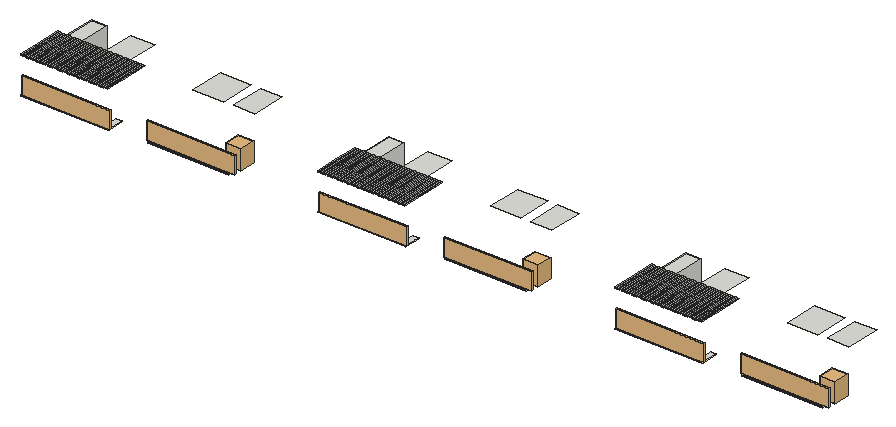
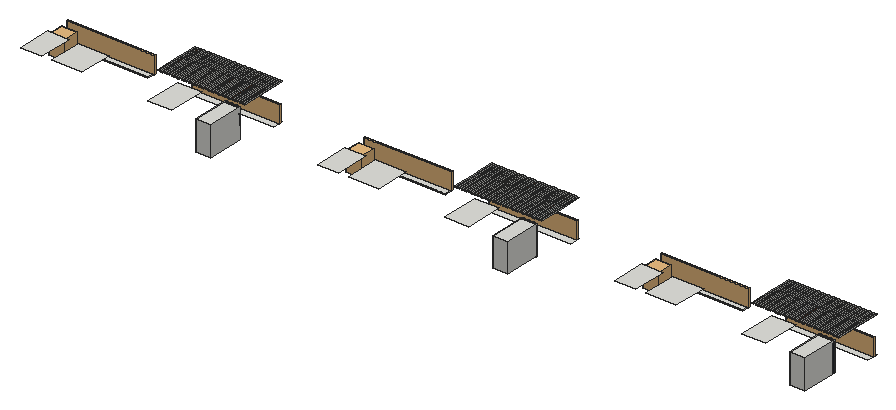
# SketchUp Ruby script. Lengths in inches.
U = 1.inch
M = Sketchup.active_model
def pt(a) = Geom::Point3d.new(a.map { |v| v * U })
def face(e, loops, mat)
  f = e.add_face(loops[0].map { |a| pt(a) })
  loops[1..].each { |l| e.add_face(l.map { |a| pt(a) }).erase! }
  f.material = f.back_material = mat if mat
  f
end
# faces: each face lists its corners as indices into pts; further lists are holes
def faces(e, pts, list, mat = nil) = list.each { |f| face(e, (f[0].is_a?(Array) ? f : [f]).map { |l| l.map { |i| pts[i] } }, mat) }
# xy, xz, yz: faces in a plane at the given z, y or x. An outline is a flat list of corners, or four numbers for a rectangle; further outlines are holes
def ring(l) = l.size == 4 ? [[l[0], l[1]], [l[2], l[1]], [l[2], l[3]], [l[0], l[3]]] : l.each_slice(2).to_a
def flat(e, list, mat, &to3) = list.each { |f| face(e, (f[0].is_a?(Array) ? f : [f]).map { |l| ring(l).map { |u, v| to3.(u, v) } }, mat) }
def xy(e, z, list, mat = nil) = flat(e, list, mat) { |x, y| [x, y, z] }
def xz(e, y, list, mat = nil) = flat(e, list, mat) { |x, z| [x, y, z] }
def yz(e, x, list, mat = nil) = flat(e, list, mat) { |y, z| [x, y, z] }
def lines(e, pts, list) = list.each { |a, b| e.add_line(pt(pts[a]), pt(pts[b])) }
# prism: a flat outline (further loops are holes) pulled along v
def prism(e, loops, v, mat = nil)
  f = face(e, loops, mat); d = Geom::Vector3d.new(v.map { |x| x * U })
  f.pushpull(f.normal.samedirection?(d) ? d.length : -d.length)
end
def box(e, o, s, mat = nil) = prism(e, [[o, [o[0] + s[0], o[1], o[2]], [o[0] + s[0], o[1] + s[1], o[2]], [o[0], o[1] + s[1], o[2]]]], [0, 0, s[2]], mat)
def at(x, y, z, deg = 0) = Geom::Transformation.translation(pt([x, y, z])) * Geom::Transformation.rotation(ORIGIN, Z_AXIS, deg.degrees)
def axes(o, x, y, z) = Geom::Transformation.new([*x, 0, *y, 0, *z, 0, *pt(o).to_a, 1])
def part(name) = M.definitions.add(name)
# library, detail: a bought-in or finely detailed component or shape, given as its bounding box
def library(name, o, s) = part(name).tap { |d| box(d.entities, o, s) }
def detail(e, o, s) = box(e.add_group.entities, o, s)
def put(e, d, t, mat = nil) = e.add_instance(d, t).tap { |i| i.material = mat if mat }
def group(e, t, mat = nil) = e.add_group.tap { |g| g.transformation = t; g.material = mat if mat }.entities
root = M.entities
M.materials.add("Wine2").color = [0, 0, 0]
M.materials["Wine2"].alpha = 0
M.materials.add("[0130_Gainsboro]").color = [39, 45, 50]
M.materials.add("[Wood Veneer 01]").color = [51, 28, 15]
c1 = library("plant (1)",[-35.72,-28.42,0],[66.31,67.39,84.38])
c2 = library("Glass Railing",[0,0,0],[139.5,4.76,42])
c3 = part("Group\#55")
xy(c3.entities,0,[[0,-0.98,43.07,0],[0,0,43.07,1.4]],"[0130_Gainsboro]")
xy(c3.entities,0.3,[[0.3,-1.43,42.77,-0.98]],"[0130_Gainsboro]")
xy(c3.entities,2.95,[[2.95,-1.43,40.12,-0.63],[2.95,-0.63,40.12,0],[2.95,0,40.12,0.64],[2.95,0.64,40.12,1.4]],"[0130_Gainsboro]")
xy(c3.entities,3.54,[[3.54,-0.63,39.53,0],[3.54,0,39.53,0.64]],"[0130_Gainsboro]")
xy(c3.entities,111.8125,[[3.54,-0.63,39.53,0],[3.54,0,39.53,0.64]],"[0130_Gainsboro]")
xy(c3.entities,112.4,[[2.95,-1.43,40.12,-0.63],[2.95,-0.63,40.12,0],[2.95,0,40.12,0.64],[2.95,0.64,40.12,1.4]],"[0130_Gainsboro]")
xy(c3.entities,115.05,[[0.3,-1.43,42.77,-0.98]],"[0130_Gainsboro]")
xy(c3.entities,115.35,[[0,-0.98,43.07,0],[0,0,43.07,1.4]],"[0130_Gainsboro]")
xz(c3.entities,-1.43,[[[0.3,0.3,42.77,115.05],[2.95,2.95,40.12,112.4]]],"[Wood Veneer 01]")
xz(c3.entities,-0.98,[[[0,0,43.07,115.35],[0.3,0.3,42.77,115.05]]],"[0130_Gainsboro]")
xz(c3.entities,-0.63,[[[2.95,2.95,40.12,112.4],[3.54,3.54,39.53,111.8125]]],"[0130_Gainsboro]")
xz(c3.entities,0,[[3.54,3.54,39.53,111.8125]],"Wine2")
xz(c3.entities,0,[[[0,0,43.07,115.35],[2.95,2.95,40.12,112.4]],[[2.95,2.95,40.12,112.4],[3.54,3.54,39.53,111.8125]]],"[0130_Gainsboro]")
xz(c3.entities,0.64,[[[2.95,2.95,40.12,112.4],[3.54,3.54,39.53,111.8125]]],"[0130_Gainsboro]")
xz(c3.entities,1.4,[[[0,0,43.07,115.35],[2.95,2.95,40.12,112.4]]],"[0130_Gainsboro]")
yz(c3.entities,0,[[-0.98,0,0,115.35],[0,0,1.4,115.35]],"[0130_Gainsboro]")
yz(c3.entities,0.3,[[-1.43,0.3,-0.98,115.05]],"[0130_Gainsboro]")
yz(c3.entities,2.95,[[-1.43,2.95,-0.63,112.4],[-0.63,2.95,0,112.4],[0,2.95,0.64,112.4],[0.64,2.95,1.4,112.4]],"[0130_Gainsboro]")
yz(c3.entities,3.54,[[-0.63,3.54,0,111.8125],[0,3.54,0.64,111.8125]],"[0130_Gainsboro]")
yz(c3.entities,39.53,[[-0.63,3.54,0,111.8125],[0,3.54,0.64,111.8125]],"[0130_Gainsboro]")
yz(c3.entities,40.12,[[-1.43,2.95,-0.63,112.4],[-0.63,2.95,0,112.4],[0,2.95,0.64,112.4],[0.64,2.95,1.4,112.4]],"[0130_Gainsboro]")
yz(c3.entities,42.77,[[-1.43,0.3,-0.98,115.05]],"[0130_Gainsboro]")
yz(c3.entities,43.07,[[-0.98,0,0,115.35],[0,0,1.4,115.35]],"[0130_Gainsboro]")
c4 = part("Component\#21")
put(c4.entities,c3,axes([90.57,1.43,0],[1.05148,0,0],[0,1,0],[0,0,1]))
put(c4.entities,c3,axes([0,1.43,0],[1.05148,0,0],[0,1,0],[0,0,1]))
put(c4.entities,c3,axes([45.29,1.43,0],[1.05148,0,0],[0,1,0],[0,0,1]),"[Wood Veneer 01]")
xy(root,289.1875,[[100.18,246.64,315.43,249.27],[315.43,246.64,318.0625,249.27],[833.74,246.64,1049,249.27],[1049,246.64,1051.625,249.27],[1567.3,246.64,1782.56,249.27],
  [1782.56,246.64,1785.1875,249.27],[100.18,249.27,315.43,249.27,315.43,290.02,301.9,290.02,301.9,271.8,100.18,271.8],[315.43,249.27,318.0625,286.21],[833.74,249.27,1049,249.27,1049,290.02,1035.46,290.02,1035.46,271.8,833.74,271.8],[1049,249.27,1051.625,286.21],
  [1567.3,249.27,1782.56,249.27,1782.56,290.02,1769.03,290.02,1769.03,271.8,1567.3,271.8],[1782.56,249.27,1785.1875,286.21]])
xy(root,290.375,[[409.32,253.22,409.32,253.84,413.01,253.84,413.01,255.84,609.07,255.84,609.07,253.22],[1142.89,253.22,1142.89,253.84,1146.57,253.84,1146.57,255.84,1342.64,255.84,1342.64,253.22],[1876.45,253.22,1876.45,253.84,1880.14,253.84,1880.14,255.84,2076.2,255.84,2076.2,253.22],[409.32,253.84,413.01,255.47],[1142.89,253.84,1146.57,255.47],
  [1876.45,253.84,1880.14,255.47],[409.32,255.47,413.01,255.84],[1142.89,255.47,1146.57,255.84],[1876.45,255.47,1880.14,255.84],[409.32,255.84,609.07,273.33],
  [1142.89,255.84,1342.64,273.33],[1876.45,255.84,2076.2,273.33]])
xy(root,292.5625,[[409.32,253.22,609.07,255.84],[1142.89,253.22,1342.64,255.84],[1876.45,253.22,2076.2,255.84],[409.32,255.84,609.07,273.33],[1142.89,255.84,1342.64,273.33],
  [1876.45,255.84,2076.2,273.33]])
xy(root,297.24,[[111.92,361.27,149.24,452.58],[845.49,361.27,882.8,452.58],[1579.05,361.27,1616.36,452.58]])
xy(root,369.36,[[207.81,361.27,266.47,452.64],[941.37,361.27,1000.03,452.64],[1674.93,361.27,1733.6,452.64]])
xy(root,369.37,[[111.92,361.27,149.24,452.58],[845.49,361.27,882.8,452.58],[1579.05,361.27,1616.36,452.58]])
xy(root,369.625,[[435.49,361.27,509.74,445.08],[1169.05,361.27,1243.3,445.08],[1902.61,361.27,1976.86,445.08]])
xy(root,369.6875,[[534.92,361.27,587.67,445.08],[1268.48,361.27,1321.23,445.08],[2002.05,361.27,2054.8,445.08]])
xy(root,378.875,[[100.18,246.64,105.12,361.27],[108.49,246.64,113.53,361.27],[116.9,246.64,121.94,361.27],[125.32,246.64,130.35,361.27],[133.73,246.64,138.77,361.27],
  [142.14,246.64,147.18,361.27],[150.55,246.64,155.59,361.27],[158.97,246.64,164.01,361.27],[167.38,246.64,172.42,361.27],[175.79,246.64,180.83,361.27],
  [184.21,246.64,189.24,361.27],[192.62,246.64,197.66,361.27],[201.03,246.64,206.07,361.27],[209.44,246.64,214.48,361.27],[217.86,246.64,222.89,361.27],
  [226.27,246.64,231.31,361.27],[234.68,246.64,239.72,361.27],[243.1,246.64,248.13,361.27],[251.51,246.64,256.55,361.27],[259.92,246.64,264.96,361.27],
  [268.33,246.64,273.37,361.27],[276.75,246.64,281.78,361.27],[285.16,246.64,290.2,361.27],[293.57,246.64,298.61,361.27],[301.98,246.64,307.02,361.27],
  [310.4,246.64,315.43,361.27],[833.74,246.64,838.68,361.27],[842.05,246.64,847.09,361.27],[850.47,246.64,855.5,361.27],[858.88,246.64,863.92,361.27],
  [867.29,246.64,872.33,361.27],[875.7,246.64,880.74,361.27],[884.12,246.64,889.16,361.27],[892.53,246.64,897.57,361.27],[900.94,246.64,905.98,361.27],
  [909.36,246.64,914.39,361.27],[917.77,246.64,922.81,361.27],[926.18,246.64,931.22,361.27],[934.59,246.64,939.63,361.27],[943.01,246.64,948.04,361.27],
  [951.42,246.64,956.46,361.27],[959.83,246.64,964.87,361.27],[968.24,246.64,973.28,361.27],[976.66,246.64,981.7,361.27],[985.07,246.64,990.11,361.27],
  [993.48,246.64,998.52,361.27],[1001.9,246.64,1006.93,361.27],[1010.31,246.64,1015.35,361.27],[1018.72,246.64,1023.76,361.27],[1027.13,246.64,1032.17,361.27],
  [1035.55,246.64,1040.58,361.27],[1043.96,246.64,1049,361.27],[1567.3,246.64,1572.24,361.27],[1575.62,246.64,1580.65,361.27],[1584.03,246.64,1589.07,361.27],
  [1592.44,246.64,1597.48,361.27],[1600.85,246.64,1605.89,361.27],[1609.27,246.64,1614.3,361.27],[1617.68,246.64,1622.72,361.27],[1626.09,246.64,1631.13,361.27],
  [1634.51,246.64,1639.54,361.27],[1642.92,246.64,1647.96,361.27],[1651.33,246.64,1656.37,361.27],[1659.74,246.64,1664.78,361.27],[1668.16,246.64,1673.19,361.27],
  [1676.57,246.64,1681.61,361.27],[1684.98,246.64,1690.02,361.27],[1693.39,246.64,1698.43,361.27],[1701.81,246.64,1706.85,361.27],[1710.22,246.64,1715.26,361.27],
  [1718.63,246.64,1723.67,361.27],[1727.05,246.64,1732.08,361.27],[1735.46,246.64,1740.5,361.27],[1743.87,246.64,1748.91,361.27],[1752.28,246.64,1757.32,361.27],
  [1760.7,246.64,1765.73,361.27],[1769.11,246.64,1774.15,361.27],[1777.52,246.64,1782.56,361.27]],"[Wood Veneer 01]")
xz(root,246.64,[[100.18,378.875,105.12,380.6875],[108.49,378.875,113.53,380.6875],[116.9,378.875,121.94,380.6875],[125.32,378.875,130.35,380.9375],[133.73,378.875,138.77,380.6875],
  [142.14,378.875,147.18,380.6875],[150.55,378.875,155.59,380.6875],[158.97,378.875,164.01,380.6875],[167.38,378.875,172.42,380.6875],[175.79,378.875,180.83,380.6875],
  [184.21,378.875,189.24,380.6875],[192.62,378.875,197.66,380.6875],[201.03,378.875,206.07,380.6875],[209.44,378.875,214.48,380.6875],[217.86,378.875,222.89,380.6875],
  [226.27,378.875,231.31,380.6875],[234.68,378.875,239.72,380.6875],[243.1,378.875,248.13,380.6875],[251.51,378.875,256.55,380.6875],[259.92,378.875,264.96,380.6875],
  [268.33,378.875,273.37,380.6875],[276.75,378.875,281.78,380.6875],[285.16,378.875,290.2,380.6875],[293.57,378.875,298.61,380.6875],[301.98,378.875,307.02,380.6875],
  [310.4,378.875,315.43,380.6875],[833.74,378.875,838.68,380.6875],[842.05,378.875,847.09,380.6875],[850.47,378.875,855.5,380.6875],[858.88,378.875,863.92,380.9375],
  [867.29,378.875,872.33,380.6875],[875.7,378.875,880.74,380.6875],[884.12,378.875,889.16,380.6875],[892.53,378.875,897.57,380.6875],[900.94,378.875,905.98,380.6875],
  [909.36,378.875,914.39,380.6875],[917.77,378.875,922.81,380.6875],[926.18,378.875,931.22,380.6875],[934.59,378.875,939.63,380.6875],[943.01,378.875,948.04,380.6875],
  [951.42,378.875,956.46,380.6875],[959.83,378.875,964.87,380.6875],[968.24,378.875,973.28,380.6875],[976.66,378.875,981.7,380.6875],[985.07,378.875,990.11,380.6875],
  [993.48,378.875,998.52,380.6875],[1001.9,378.875,1006.93,380.6875],[1010.31,378.875,1015.35,380.6875],[1018.72,378.875,1023.76,380.6875],[1027.13,378.875,1032.17,380.6875],
  [1035.55,378.875,1040.58,380.6875],[1043.96,378.875,1049,380.6875],[1567.3,378.875,1572.24,380.6875],[1575.62,378.875,1580.65,380.6875],[1584.03,378.875,1589.07,380.6875],
  [1592.44,378.875,1597.48,380.9375],[1600.85,378.875,1605.89,380.6875],[1609.27,378.875,1614.3,380.6875],[1617.68,378.875,1622.72,380.6875],[1626.09,378.875,1631.13,380.6875],
  [1634.51,378.875,1639.54,380.6875],[1642.92,378.875,1647.96,380.6875],[1651.33,378.875,1656.37,380.6875],[1659.74,378.875,1664.78,380.6875],[1668.16,378.875,1673.19,380.6875],
  [1676.57,378.875,1681.61,380.6875],[1684.98,378.875,1690.02,380.6875],[1693.39,378.875,1698.43,380.6875],[1701.81,378.875,1706.85,380.6875],[1710.22,378.875,1715.26,380.6875],
  [1718.63,378.875,1723.67,380.6875],[1727.05,378.875,1732.08,380.6875],[1735.46,378.875,1740.5,380.6875],[1743.87,378.875,1748.91,380.6875],[1752.28,378.875,1757.32,380.6875],
  [1760.7,378.875,1765.73,380.6875],[1769.11,378.875,1774.15,380.6875],[1777.52,378.875,1782.56,380.6875]],"[Wood Veneer 01]")
xz(root,253.22,[[409.32,290.375,609.07,292.5625],[1142.89,290.375,1342.64,292.5625],[1876.45,290.375,2076.2,292.5625]],"[Wood Veneer 01]")
xz(root,255.84,[[409.32,290.375,609.07,292.5625],[1142.89,290.375,1342.64,292.5625],[1876.45,290.375,2076.2,292.5625]])
xz(root,273.33,[[409.32,290.375,609.07,292.5625],[1142.89,290.375,1342.64,292.5625],[1876.45,290.375,2076.2,292.5625]])
xz(root,361.27,[[100.18,378.875,105.12,380.6875],[108.49,378.875,113.53,380.6875],[116.9,378.875,121.94,380.6875],[125.32,378.875,130.35,380.9375],[133.73,378.875,138.77,380.6875],
  [142.14,378.875,147.18,380.6875],[150.55,378.875,155.59,380.6875],[158.97,378.875,164.01,380.6875],[167.38,378.875,172.42,380.6875],[175.79,378.875,180.83,380.6875],
  [184.21,378.875,189.24,380.6875],[192.62,378.875,197.66,380.6875],[201.03,378.875,206.07,380.6875],[209.44,378.875,214.48,380.6875],[217.86,378.875,222.89,380.6875],
  [226.27,378.875,231.31,380.6875],[234.68,378.875,239.72,380.6875],[243.1,378.875,248.13,380.6875],[251.51,378.875,256.55,380.6875],[259.92,378.875,264.96,380.6875],
  [268.33,378.875,273.37,380.6875],[276.75,378.875,281.78,380.6875],[285.16,378.875,290.2,380.6875],[293.57,378.875,298.61,380.6875],[301.98,378.875,307.02,380.6875],
  [310.4,378.875,315.43,380.6875],[833.74,378.875,838.68,380.6875],[842.05,378.875,847.09,380.6875],[850.47,378.875,855.5,380.6875],[858.88,378.875,863.92,380.9375],
  [867.29,378.875,872.33,380.6875],[875.7,378.875,880.74,380.6875],[884.12,378.875,889.16,380.6875],[892.53,378.875,897.57,380.6875],[900.94,378.875,905.98,380.6875],
  [909.36,378.875,914.39,380.6875],[917.77,378.875,922.81,380.6875],[926.18,378.875,931.22,380.6875],[934.59,378.875,939.63,380.6875],[943.01,378.875,948.04,380.6875],
  [951.42,378.875,956.46,380.6875],[959.83,378.875,964.87,380.6875],[968.24,378.875,973.28,380.6875],[976.66,378.875,981.7,380.6875],[985.07,378.875,990.11,380.6875],
  [993.48,378.875,998.52,380.6875],[1001.9,378.875,1006.93,380.6875],[1010.31,378.875,1015.35,380.6875],[1018.72,378.875,1023.76,380.6875],[1027.13,378.875,1032.17,380.6875],
  [1035.55,378.875,1040.58,380.6875],[1043.96,378.875,1049,380.6875],[1567.3,378.875,1572.24,380.6875],[1575.62,378.875,1580.65,380.6875],[1584.03,378.875,1589.07,380.6875],
  [1592.44,378.875,1597.48,380.9375],[1600.85,378.875,1605.89,380.6875],[1609.27,378.875,1614.3,380.6875],[1617.68,378.875,1622.72,380.6875],[1626.09,378.875,1631.13,380.6875],
  [1634.51,378.875,1639.54,380.6875],[1642.92,378.875,1647.96,380.6875],[1651.33,378.875,1656.37,380.6875],[1659.74,378.875,1664.78,380.6875],[1668.16,378.875,1673.19,380.6875],
  [1676.57,378.875,1681.61,380.6875],[1684.98,378.875,1690.02,380.6875],[1693.39,378.875,1698.43,380.6875],[1701.81,378.875,1706.85,380.6875],[1710.22,378.875,1715.26,380.6875],
  [1718.63,378.875,1723.67,380.6875],[1727.05,378.875,1732.08,380.6875],[1735.46,378.875,1740.5,380.6875],[1743.87,378.875,1748.91,380.6875],[1752.28,378.875,1757.32,380.6875],
  [1760.7,378.875,1765.73,380.6875],[1769.11,378.875,1774.15,380.6875],[1777.52,378.875,1782.56,380.6875]])
xz(root,452.58,[[111.92,297.24,149.24,369.37],[845.49,297.24,882.8,369.37],[1579.05,297.24,1616.36,369.37]])
yz(root,100.18,[[246.64,378.875,293.45,380.6875],[293.45,378.875,293.46,380.6875],[293.46,378.875,361.27,380.6875]])
yz(root,105.12,[[246.64,378.875,286.21,380.6875],[286.21,378.875,293.45,380.6875],[293.45,378.875,361.27,380.6875]])
yz(root,108.49,[[246.64,378.875,361.27,380.6875]])
yz(root,111.92,[[361.27,297.24,452.58,369.37]])
yz(root,113.53,[[246.64,378.875,286.21,380.6875],[286.21,378.875,293.45,380.6875],[293.45,378.875,361.27,380.6875]])
yz(root,116.9,[[246.64,378.875,361.27,380.6875]])
yz(root,121.94,[[246.64,378.875,286.21,380.6875],[286.21,378.875,293.45,380.6875],[293.45,378.875,361.27,380.6875]])
yz(root,125.32,[[246.64,378.875,361.27,380.6875]])
yz(root,130.35,[[246.64,378.875,286.21,380.6875],[286.21,378.875,293.45,380.6875],[293.45,378.875,361.27,380.6875]])
yz(root,133.73,[[246.64,378.875,361.27,380.6875]])
yz(root,138.77,[[246.64,378.875,286.21,380.6875],[286.21,378.875,293.45,380.6875],[293.45,378.875,361.27,380.6875]])
yz(root,142.14,[[246.64,378.875,361.27,380.6875]])
yz(root,147.18,[[246.64,378.875,286.21,380.6875],[286.21,378.875,293.45,380.6875],[293.45,378.875,361.27,380.6875]])
yz(root,149.24,[[361.27,297.24,452.58,369.37]])
yz(root,150.55,[[246.64,378.875,361.27,380.6875]])
yz(root,155.59,[[246.64,378.875,286.21,380.6875],[286.21,378.875,293.45,380.6875],[293.45,378.875,361.27,380.6875]])
yz(root,158.97,[[246.64,378.875,361.27,380.6875]])
yz(root,164.01,[[246.64,378.875,286.21,380.6875],[286.21,378.875,293.45,380.6875],[293.45,378.875,361.27,380.6875]])
yz(root,167.38,[[246.64,378.875,361.27,380.6875]])
yz(root,172.42,[[246.64,378.875,286.21,380.6875],[286.21,378.875,293.45,380.6875],[293.45,378.875,361.27,380.6875]])
yz(root,175.79,[[246.64,378.875,361.27,380.6875]])
yz(root,180.83,[[246.64,378.875,286.21,380.6875],[286.21,378.875,293.45,380.6875],[293.45,378.875,361.27,380.6875]])
yz(root,184.21,[[246.64,378.875,361.27,380.6875]])
yz(root,189.24,[[246.64,378.875,286.21,380.6875],[286.21,378.875,293.45,380.6875],[293.45,378.875,361.27,380.6875]])
yz(root,192.62,[[246.64,378.875,361.27,380.6875]])
yz(root,197.66,[[246.64,378.875,286.21,380.6875],[286.21,378.875,293.45,380.6875],[293.45,378.875,361.27,380.6875]])
yz(root,201.03,[[246.64,378.875,361.27,380.6875]])
yz(root,206.07,[[246.64,378.875,286.21,380.6875],[286.21,378.875,293.45,380.6875],[293.45,378.875,361.27,380.6875]])
yz(root,209.44,[[246.64,378.875,361.27,380.6875]])
yz(root,214.48,[[246.64,378.875,286.21,380.6875],[286.21,378.875,293.45,380.6875],[293.45,378.875,361.27,380.6875]])
yz(root,217.86,[[246.64,378.875,361.27,380.6875]])
yz(root,222.89,[[246.64,378.875,286.21,380.6875],[286.21,378.875,293.45,380.6875],[293.45,378.875,361.27,380.6875]])
yz(root,226.27,[[246.64,378.875,361.27,380.6875]])
yz(root,231.31,[[246.64,378.875,286.21,380.6875],[286.21,378.875,293.45,380.6875],[293.45,378.875,361.27,380.6875]])
yz(root,234.68,[[246.64,378.875,361.27,380.6875]])
yz(root,239.72,[[246.64,378.875,286.21,380.6875],[286.21,378.875,293.45,380.6875],[293.45,378.875,361.27,380.6875]])
yz(root,243.1,[[246.64,378.875,361.27,380.6875]])
yz(root,248.13,[[246.64,378.875,286.21,380.6875],[286.21,378.875,293.45,380.6875],[293.45,378.875,361.27,380.6875]])
yz(root,251.51,[[246.64,378.875,361.27,380.6875]])
yz(root,256.55,[[246.64,378.875,286.21,380.6875],[286.21,378.875,293.45,380.6875],[293.45,378.875,361.27,380.6875]])
yz(root,259.92,[[246.64,378.875,361.27,380.6875]])
yz(root,264.96,[[246.64,378.875,286.21,380.6875],[286.21,378.875,293.45,380.6875],[293.45,378.875,361.27,380.6875]])
yz(root,268.33,[[246.64,378.875,361.27,380.6875]])
yz(root,273.37,[[246.64,378.875,286.21,380.6875],[286.21,378.875,293.45,380.6875],[293.45,378.875,361.27,380.6875]])
yz(root,276.75,[[246.64,378.875,361.27,380.6875]])
yz(root,281.78,[[246.64,378.875,286.21,380.6875],[286.21,378.875,293.45,380.6875],[293.45,378.875,361.27,380.6875]])
yz(root,285.16,[[246.64,378.875,361.27,380.6875]])
yz(root,290.2,[[246.64,378.875,286.21,380.6875],[286.21,378.875,293.45,380.6875],[293.45,378.875,361.27,380.6875]])
yz(root,293.57,[[246.64,378.875,361.27,380.6875]])
yz(root,298.61,[[246.64,378.875,286.21,380.6875],[286.21,378.875,293.45,380.6875],[293.45,378.875,361.27,380.6875]])
yz(root,301.98,[[246.64,378.875,361.27,380.6875]])
yz(root,307.02,[[246.64,378.875,286.21,380.6875],[286.21,378.875,293.45,380.6875],[293.45,378.875,361.27,380.6875]])
yz(root,310.4,[[246.64,378.875,361.27,380.6875]])
yz(root,315.43,[[246.64,378.875,286.21,380.6875],[286.21,378.875,293.45,380.6875],[293.45,378.875,361.27,380.6875]])
yz(root,409.32,[[253.22,290.375,255.84,292.5625],[255.84,290.375,273.33,292.5625]])
yz(root,609.07,[[253.22,290.375,255.84,292.5625],[255.84,290.375,273.33,292.5625]])
yz(root,833.74,[[246.64,378.875,293.45,380.6875],[293.45,378.875,293.46,380.6875],[293.46,378.875,361.27,380.6875]])
yz(root,838.68,[[246.64,378.875,286.21,380.6875],[286.21,378.875,293.45,380.6875],[293.45,378.875,361.27,380.6875]])
yz(root,842.05,[[246.64,378.875,361.27,380.6875]])
yz(root,845.49,[[361.27,297.24,452.58,369.37]])
yz(root,847.09,[[246.64,378.875,286.21,380.6875],[286.21,378.875,293.45,380.6875],[293.45,378.875,361.27,380.6875]])
yz(root,850.47,[[246.64,378.875,361.27,380.6875]])
yz(root,855.5,[[246.64,378.875,286.21,380.6875],[286.21,378.875,293.45,380.6875],[293.45,378.875,361.27,380.6875]])
yz(root,858.88,[[246.64,378.875,361.27,380.6875]])
yz(root,863.92,[[246.64,378.875,286.21,380.6875],[286.21,378.875,293.45,380.6875],[293.45,378.875,361.27,380.6875]])
yz(root,867.29,[[246.64,378.875,361.27,380.6875]])
yz(root,872.33,[[246.64,378.875,286.21,380.6875],[286.21,378.875,293.45,380.6875],[293.45,378.875,361.27,380.6875]])
yz(root,875.7,[[246.64,378.875,361.27,380.6875]])
yz(root,880.74,[[246.64,378.875,286.21,380.6875],[286.21,378.875,293.45,380.6875],[293.45,378.875,361.27,380.6875]])
yz(root,882.8,[[361.27,297.24,452.58,369.37]])
yz(root,884.12,[[246.64,378.875,361.27,380.6875]])
yz(root,889.16,[[246.64,378.875,286.21,380.6875],[286.21,378.875,293.45,380.6875],[293.45,378.875,361.27,380.6875]])
yz(root,892.53,[[246.64,378.875,361.27,380.6875]])
yz(root,897.57,[[246.64,378.875,286.21,380.6875],[286.21,378.875,293.45,380.6875],[293.45,378.875,361.27,380.6875]])
yz(root,900.94,[[246.64,378.875,361.27,380.6875]])
yz(root,905.98,[[246.64,378.875,286.21,380.6875],[286.21,378.875,293.45,380.6875],[293.45,378.875,361.27,380.6875]])
yz(root,909.36,[[246.64,378.875,361.27,380.6875]])
yz(root,914.39,[[246.64,378.875,286.21,380.6875],[286.21,378.875,293.45,380.6875],[293.45,378.875,361.27,380.6875]])
yz(root,917.77,[[246.64,378.875,361.27,380.6875]])
yz(root,922.81,[[246.64,378.875,286.21,380.6875],[286.21,378.875,293.45,380.6875],[293.45,378.875,361.27,380.6875]])
yz(root,926.18,[[246.64,378.875,361.27,380.6875]])
yz(root,931.22,[[246.64,378.875,286.21,380.6875],[286.21,378.875,293.45,380.6875],[293.45,378.875,361.27,380.6875]])
yz(root,934.59,[[246.64,378.875,361.27,380.6875]])
yz(root,939.63,[[246.64,378.875,286.21,380.6875],[286.21,378.875,293.45,380.6875],[293.45,378.875,361.27,380.6875]])
yz(root,943.01,[[246.64,378.875,361.27,380.6875]])
yz(root,948.04,[[246.64,378.875,286.21,380.6875],[286.21,378.875,293.45,380.6875],[293.45,378.875,361.27,380.6875]])
yz(root,951.42,[[246.64,378.875,361.27,380.6875]])
yz(root,956.46,[[246.64,378.875,286.21,380.6875],[286.21,378.875,293.45,380.6875],[293.45,378.875,361.27,380.6875]])
yz(root,959.83,[[246.64,378.875,361.27,380.6875]])
yz(root,964.87,[[246.64,378.875,286.21,380.6875],[286.21,378.875,293.45,380.6875],[293.45,378.875,361.27,380.6875]])
yz(root,968.24,[[246.64,378.875,361.27,380.6875]])
yz(root,973.28,[[246.64,378.875,286.21,380.6875],[286.21,378.875,293.45,380.6875],[293.45,378.875,361.27,380.6875]])
yz(root,976.66,[[246.64,378.875,361.27,380.6875]])
yz(root,981.7,[[246.64,378.875,286.21,380.6875],[286.21,378.875,293.45,380.6875],[293.45,378.875,361.27,380.6875]])
yz(root,985.07,[[246.64,378.875,361.27,380.6875]])
yz(root,990.11,[[246.64,378.875,286.21,380.6875],[286.21,378.875,293.45,380.6875],[293.45,378.875,361.27,380.6875]])
yz(root,993.48,[[246.64,378.875,361.27,380.6875]])
yz(root,998.52,[[246.64,378.875,286.21,380.6875],[286.21,378.875,293.45,380.6875],[293.45,378.875,361.27,380.6875]])
yz(root,1001.9,[[246.64,378.875,361.27,380.6875]])
yz(root,1006.93,[[246.64,378.875,286.21,380.6875],[286.21,378.875,293.45,380.6875],[293.45,378.875,361.27,380.6875]])
yz(root,1010.31,[[246.64,378.875,361.27,380.6875]])
yz(root,1015.35,[[246.64,378.875,286.21,380.6875],[286.21,378.875,293.45,380.6875],[293.45,378.875,361.27,380.6875]])
yz(root,1018.72,[[246.64,378.875,361.27,380.6875]])
yz(root,1023.76,[[246.64,378.875,286.21,380.6875],[286.21,378.875,293.45,380.6875],[293.45,378.875,361.27,380.6875]])
yz(root,1027.13,[[246.64,378.875,361.27,380.6875]])
yz(root,1032.17,[[246.64,378.875,286.21,380.6875],[286.21,378.875,293.45,380.6875],[293.45,378.875,361.27,380.6875]])
yz(root,1035.55,[[246.64,378.875,361.27,380.6875]])
yz(root,1040.58,[[246.64,378.875,286.21,380.6875],[286.21,378.875,293.45,380.6875],[293.45,378.875,361.27,380.6875]])
yz(root,1043.96,[[246.64,378.875,361.27,380.6875]])
yz(root,1049,[[246.64,378.875,286.21,380.6875],[286.21,378.875,293.45,380.6875],[293.45,378.875,361.27,380.6875]])
yz(root,1142.89,[[253.22,290.375,255.84,292.5625],[255.84,290.375,273.33,292.5625]])
yz(root,1342.64,[[253.22,290.375,255.84,292.5625],[255.84,290.375,273.33,292.5625]])
yz(root,1567.3,[[246.64,378.875,293.45,380.6875],[293.45,378.875,293.46,380.6875],[293.46,378.875,361.27,380.6875]])
yz(root,1572.24,[[246.64,378.875,286.21,380.6875],[286.21,378.875,293.45,380.6875],[293.45,378.875,361.27,380.6875]])
yz(root,1575.62,[[246.64,378.875,361.27,380.6875]])
yz(root,1579.05,[[361.27,297.24,452.58,369.37]])
yz(root,1580.65,[[246.64,378.875,286.21,380.6875],[286.21,378.875,293.45,380.6875],[293.45,378.875,361.27,380.6875]])
yz(root,1584.03,[[246.64,378.875,361.27,380.6875]])
yz(root,1589.07,[[246.64,378.875,286.21,380.6875],[286.21,378.875,293.45,380.6875],[293.45,378.875,361.27,380.6875]])
yz(root,1592.44,[[246.64,378.875,361.27,380.6875]])
yz(root,1597.48,[[246.64,378.875,286.21,380.6875],[286.21,378.875,293.45,380.6875],[293.45,378.875,361.27,380.6875]])
yz(root,1600.85,[[246.64,378.875,361.27,380.6875]])
yz(root,1605.89,[[246.64,378.875,286.21,380.6875],[286.21,378.875,293.45,380.6875],[293.45,378.875,361.27,380.6875]])
yz(root,1609.27,[[246.64,378.875,361.27,380.6875]])
yz(root,1614.3,[[246.64,378.875,286.21,380.6875],[286.21,378.875,293.45,380.6875],[293.45,378.875,361.27,380.6875]])
yz(root,1616.36,[[361.27,297.24,452.58,369.37]])
yz(root,1617.68,[[246.64,378.875,361.27,380.6875]])
yz(root,1622.72,[[246.64,378.875,286.21,380.6875],[286.21,378.875,293.45,380.6875],[293.45,378.875,361.27,380.6875]])
yz(root,1626.09,[[246.64,378.875,361.27,380.6875]])
yz(root,1631.13,[[246.64,378.875,286.21,380.6875],[286.21,378.875,293.45,380.6875],[293.45,378.875,361.27,380.6875]])
yz(root,1634.51,[[246.64,378.875,361.27,380.6875]])
yz(root,1639.54,[[246.64,378.875,286.21,380.6875],[286.21,378.875,293.45,380.6875],[293.45,378.875,361.27,380.6875]])
yz(root,1642.92,[[246.64,378.875,361.27,380.6875]])
yz(root,1647.96,[[246.64,378.875,286.21,380.6875],[286.21,378.875,293.45,380.6875],[293.45,378.875,361.27,380.6875]])
yz(root,1651.33,[[246.64,378.875,361.27,380.6875]])
yz(root,1656.37,[[246.64,378.875,286.21,380.6875],[286.21,378.875,293.45,380.6875],[293.45,378.875,361.27,380.6875]])
yz(root,1659.74,[[246.64,378.875,361.27,380.6875]])
yz(root,1664.78,[[246.64,378.875,286.21,380.6875],[286.21,378.875,293.45,380.6875],[293.45,378.875,361.27,380.6875]])
yz(root,1668.16,[[246.64,378.875,361.27,380.6875]])
yz(root,1673.19,[[246.64,378.875,286.21,380.6875],[286.21,378.875,293.45,380.6875],[293.45,378.875,361.27,380.6875]])
yz(root,1676.57,[[246.64,378.875,361.27,380.6875]])
yz(root,1681.61,[[246.64,378.875,286.21,380.6875],[286.21,378.875,293.45,380.6875],[293.45,378.875,361.27,380.6875]])
yz(root,1684.98,[[246.64,378.875,361.27,380.6875]])
yz(root,1690.02,[[246.64,378.875,286.21,380.6875],[286.21,378.875,293.45,380.6875],[293.45,378.875,361.27,380.6875]])
yz(root,1693.39,[[246.64,378.875,361.27,380.6875]])
yz(root,1698.43,[[246.64,378.875,286.21,380.6875],[286.21,378.875,293.45,380.6875],[293.45,378.875,361.27,380.6875]])
yz(root,1701.81,[[246.64,378.875,361.27,380.6875]])
yz(root,1706.85,[[246.64,378.875,286.21,380.6875],[286.21,378.875,293.45,380.6875],[293.45,378.875,361.27,380.6875]])
yz(root,1710.22,[[246.64,378.875,361.27,380.6875]])
yz(root,1715.26,[[246.64,378.875,286.21,380.6875],[286.21,378.875,293.45,380.6875],[293.45,378.875,361.27,380.6875]])
yz(root,1718.63,[[246.64,378.875,361.27,380.6875]])
yz(root,1723.67,[[246.64,378.875,286.21,380.6875],[286.21,378.875,293.45,380.6875],[293.45,378.875,361.27,380.6875]])
yz(root,1727.05,[[246.64,378.875,361.27,380.6875]])
yz(root,1732.08,[[246.64,378.875,286.21,380.6875],[286.21,378.875,293.45,380.6875],[293.45,378.875,361.27,380.6875]])
yz(root,1735.46,[[246.64,378.875,361.27,380.6875]])
yz(root,1740.5,[[246.64,378.875,286.21,380.6875],[286.21,378.875,293.45,380.6875],[293.45,378.875,361.27,380.6875]])
yz(root,1743.87,[[246.64,378.875,361.27,380.6875]])
yz(root,1748.91,[[246.64,378.875,286.21,380.6875],[286.21,378.875,293.45,380.6875],[293.45,378.875,361.27,380.6875]])
yz(root,1752.28,[[246.64,378.875,361.27,380.6875]])
yz(root,1757.32,[[246.64,378.875,286.21,380.6875],[286.21,378.875,293.45,380.6875],[293.45,378.875,361.27,380.6875]])
yz(root,1760.7,[[246.64,378.875,361.27,380.6875]])
yz(root,1765.73,[[246.64,378.875,286.21,380.6875],[286.21,378.875,293.45,380.6875],[293.45,378.875,361.27,380.6875]])
yz(root,1769.11,[[246.64,378.875,361.27,380.6875]])
yz(root,1774.15,[[246.64,378.875,286.21,380.6875],[286.21,378.875,293.45,380.6875],[293.45,378.875,361.27,380.6875]])
yz(root,1777.52,[[246.64,378.875,361.27,380.6875]])
yz(root,1782.56,[[246.64,378.875,286.21,380.6875],[286.21,378.875,293.45,380.6875],[293.45,378.875,361.27,380.6875]])
yz(root,1876.45,[[253.22,290.375,255.84,292.5625],[255.84,290.375,273.33,292.5625]])
yz(root,2076.2,[[253.22,290.375,255.84,292.5625],[255.84,290.375,273.33,292.5625]])
p = [[833.74,249.27,289.25],[833.74,249.27,289.1875],[837.02,249.27,289.1875],[837.02,249.27,289.25],[1570.58,249.27,289.1875],[1570.58,249.27,289.25],
  [1567.3,249.27,289.25],[1567.3,249.27,289.1875],[103.45,249.27,289.1875],[103.45,249.27,289.25],[100.18,249.27,289.25],[100.18,249.27,289.1875]]
lines(root,p,[[0,1],[2,3],[4,5],[6,7],[8,9],[10,11]])
put(root,c1,axes([1332.13,298.81,288.87],[0.57,0,0],[0,0.57,0],[0,0,0.57]))
put(root,c1,axes([2065.69,298.81,288.87],[0.57,0,0],[0,0.57,0],[0,0,0.57]))
put(root,c1,axes([598.57,298.81,288.87],[0.57,0,0],[0,0.57,0],[0,0,0.57]))
put(root,c2,axes([834.26,249.55,289.1875],[1.55814,0,0],[0,1,0],[0,0,1]))
put(root,c2,axes([1567.83,249.55,289.1875],[1.55814,0,0],[0,1,0],[0,0,1]))
put(root,c2,axes([100.7,249.55,289.1875],[1.55814,0,0],[0,1,0],[0,0,1]))
put(root,c2,axes([1138.2,255.14,293.87],[1.55814,0,0],[0,1,0],[0,0,1]))
put(root,c2,axes([1871.77,255.14,293.87],[1.55814,0,0],[0,1,0],[0,0,1]))
put(root,c2,axes([404.64,255.14,293.87],[1.55814,0,0],[0,1,0],[0,0,1]))
put(root,c4,axes([845.49,361.27,297.24],[0.27464,0,0],[0,1.2771,0],[0,0,0.62578]))
put(root,c4,axes([1579.05,361.27,297.24],[0.27464,0,0],[0,1.2771,0],[0,0,0.62578]))
put(root,c4,axes([111.92,361.27,297.24],[0.27464,0,0],[0,1.2771,0],[0,0,0.62578]))
